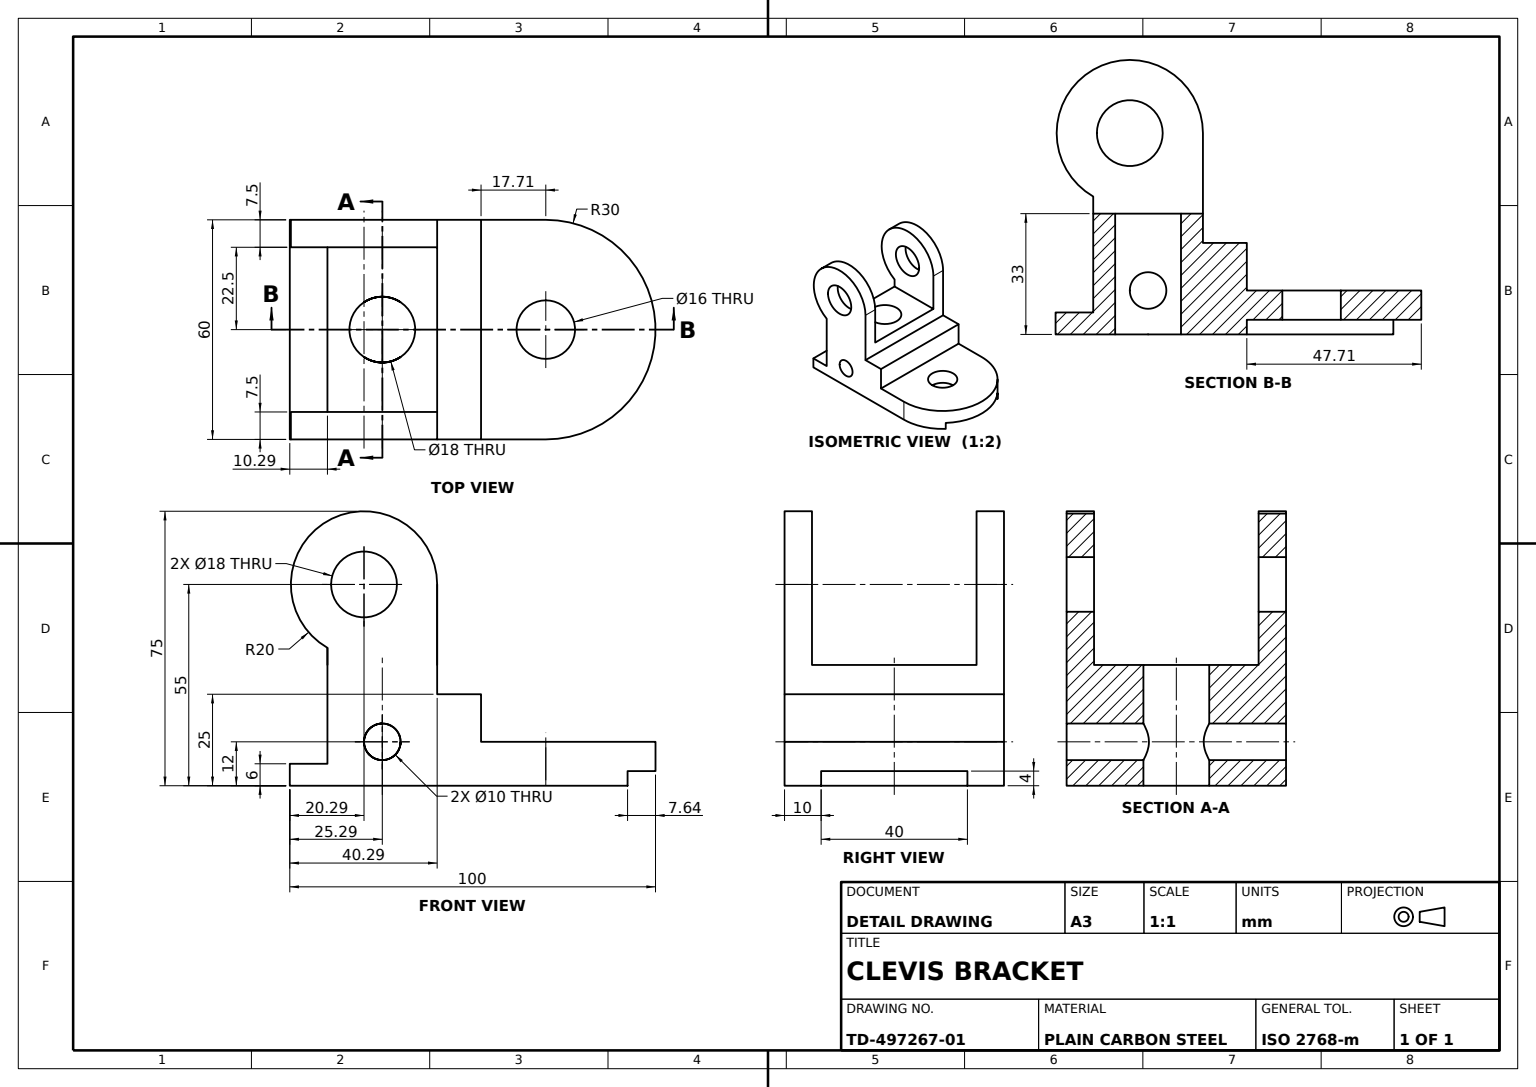
ISO-10303-21;
HEADER;
FILE_DESCRIPTION((''),'2;1');
FILE_NAME('','',(''),(''),'','','');
FILE_SCHEMA(('AUTOMOTIVE_DESIGN'));
ENDSEC;
DATA;
#1=APPLICATION_CONTEXT('');
#2=PRODUCT_CONTEXT('',#1,'mechanical');
#3=PRODUCT('','','',(#2));
#4=PRODUCT_DEFINITION_FORMATION('','',#3);
#5=PRODUCT_DEFINITION_CONTEXT('',#1,'design');
#6=PRODUCT_DEFINITION('','',#4,#5);
#7=PRODUCT_DEFINITION_SHAPE('','',#6);
#8=(LENGTH_UNIT()NAMED_UNIT(*)SI_UNIT(.MILLI.,.METRE.));
#9=(NAMED_UNIT(*)PLANE_ANGLE_UNIT()SI_UNIT($,.RADIAN.));
#10=(NAMED_UNIT(*)SI_UNIT($,.STERADIAN.)SOLID_ANGLE_UNIT());
#11=UNCERTAINTY_MEASURE_WITH_UNIT(LENGTH_MEASURE(1.E-05),#8,'distance_accuracy_value','');
#12=(GEOMETRIC_REPRESENTATION_CONTEXT(3)GLOBAL_UNCERTAINTY_ASSIGNED_CONTEXT((#11))GLOBAL_UNIT_ASSIGNED_CONTEXT((#8,#9,#10))REPRESENTATION_CONTEXT('',''));
#13=CARTESIAN_POINT('',(-9.705549,55.,-22.5));
#14=VERTEX_POINT('',#13);
#15=CARTESIAN_POINT('',(-9.705549,33.,-22.5));
#16=VERTEX_POINT('',#15);
#17=DIRECTION('',(0.,-1.,0.));
#18=VECTOR('',#17,1000.);
#19=LINE('',#13,#18);
#20=EDGE_CURVE('',#14,#16,#19,.T.);
#21=ORIENTED_EDGE('',*,*,#20,.T.);
#22=CARTESIAN_POINT('',(-9.705549,33.,22.5));
#23=VERTEX_POINT('',#22);
#24=CARTESIAN_POINT('',(-9.705549,33.,-30.));
#25=DIRECTION('',(0.,0.,1.));
#26=VECTOR('',#25,1000.);
#27=LINE('',#24,#26);
#28=EDGE_CURVE('',#16,#23,#27,.T.);
#29=ORIENTED_EDGE('',*,*,#28,.T.);
#30=CARTESIAN_POINT('',(-9.705549,55.,22.5));
#31=VERTEX_POINT('',#30);
#32=DIRECTION('',(0.,1.,0.));
#33=VECTOR('',#32,1000.);
#34=LINE('',#30,#33);
#35=EDGE_CURVE('',#23,#31,#34,.T.);
#36=ORIENTED_EDGE('',*,*,#35,.T.);
#37=CARTESIAN_POINT('',(-9.705549,55.,30.));
#38=VERTEX_POINT('',#37);
#39=LINE('',#30,#26);
#40=EDGE_CURVE('',#31,#38,#39,.T.);
#41=ORIENTED_EDGE('',*,*,#40,.T.);
#42=CARTESIAN_POINT('',(-9.705549,25.,30.));
#43=VERTEX_POINT('',#42);
#44=CARTESIAN_POINT('',(-9.705549,0.,30.));
#45=LINE('',#44,#33);
#46=EDGE_CURVE('',#43,#38,#45,.T.);
#47=ORIENTED_EDGE('',*,*,#46,.F.);
#48=CARTESIAN_POINT('',(-9.705549,25.,-30.));
#49=VERTEX_POINT('',#48);
#50=LINE('',#48,#26);
#51=EDGE_CURVE('',#49,#43,#50,.T.);
#52=ORIENTED_EDGE('',*,*,#51,.F.);
#53=CARTESIAN_POINT('',(-9.705549,55.,-30.));
#54=VERTEX_POINT('',#53);
#55=CARTESIAN_POINT('',(-9.705549,0.,-30.));
#56=LINE('',#55,#33);
#57=EDGE_CURVE('',#49,#54,#56,.T.);
#58=ORIENTED_EDGE('',*,*,#57,.T.);
#59=DIRECTION('',(0.,0.,-1.));
#60=VECTOR('',#59,1000.);
#61=LINE('',#13,#60);
#62=EDGE_CURVE('',#14,#54,#61,.T.);
#63=ORIENTED_EDGE('',*,*,#62,.F.);
#64=EDGE_LOOP('',(#21,#29,#36,#41,#47,#52,#58,#63));
#65=FACE_OUTER_BOUND('',#64,.T.);
#66=DIRECTION('',(1.,0.,0.));
#67=AXIS2_PLACEMENT_3D('',#55,#66,#59);
#68=PLANE('',#67);
#69=ADVANCED_FACE('',(#65),#68,.T.);
#70=CARTESIAN_POINT('',(2.294451,12.,30.));
#71=VERTEX_POINT('',#70);
#72=CARTESIAN_POINT('',(20.,12.,30.));
#73=VERTEX_POINT('',#72);
#74=VECTOR('',#66,1000.);
#75=LINE('',#70,#74);
#76=EDGE_CURVE('',#71,#73,#75,.T.);
#77=ORIENTED_EDGE('',*,*,#76,.T.);
#78=CARTESIAN_POINT('',(20.,12.,-30.));
#79=VERTEX_POINT('',#78);
#80=CARTESIAN_POINT('',(20.,12.,0.));
#81=AXIS2_PLACEMENT_3D('',#80,#32,#59);
#82=CIRCLE('',#81,30.);
#83=EDGE_CURVE('',#73,#79,#82,.T.);
#84=ORIENTED_EDGE('',*,*,#83,.T.);
#85=CARTESIAN_POINT('',(2.294451,12.,-30.));
#86=VERTEX_POINT('',#85);
#87=DIRECTION('',(-1.,0.,0.));
#88=VECTOR('',#87,1000.);
#89=LINE('',#78,#88);
#90=EDGE_CURVE('',#79,#86,#89,.T.);
#91=ORIENTED_EDGE('',*,*,#90,.T.);
#92=LINE('',#85,#26);
#93=EDGE_CURVE('',#86,#71,#92,.T.);
#94=ORIENTED_EDGE('',*,*,#93,.T.);
#95=EDGE_LOOP('',(#77,#84,#91,#94));
#96=FACE_OUTER_BOUND('',#95,.T.);
#97=CARTESIAN_POINT('',(20.,12.,8.));
#98=VERTEX_POINT('',#97);
#99=CARTESIAN_POINT('',(20.,12.,-8.));
#100=VERTEX_POINT('',#99);
#101=AXIS2_PLACEMENT_3D('',#80,#32,#25);
#102=CIRCLE('',#101,8.);
#103=EDGE_CURVE('',#98,#100,#102,.T.);
#104=ORIENTED_EDGE('',*,*,#103,.F.);
#105=EDGE_CURVE('',#100,#98,#102,.T.);
#106=ORIENTED_EDGE('',*,*,#105,.F.);
#107=EDGE_LOOP('',(#104,#106));
#108=FACE_BOUND('',#107,.T.);
#109=AXIS2_PLACEMENT_3D('',#80,#17,#59);
#110=PLANE('',#109);
#111=ADVANCED_FACE('',(#96,#108),#110,.F.);
#112=CARTESIAN_POINT('',(-39.705549,33.,22.5));
#113=VERTEX_POINT('',#112);
#114=LINE('',#112,#74);
#115=EDGE_CURVE('',#113,#23,#114,.T.);
#116=ORIENTED_EDGE('',*,*,#115,.T.);
#117=ORIENTED_EDGE('',*,*,#28,.F.);
#118=CARTESIAN_POINT('',(-39.705549,33.,-22.5));
#119=VERTEX_POINT('',#118);
#120=LINE('',#118,#88);
#121=EDGE_CURVE('',#16,#119,#120,.T.);
#122=ORIENTED_EDGE('',*,*,#121,.T.);
#123=CARTESIAN_POINT('',(-39.705549,33.,-30.));
#124=LINE('',#123,#26);
#125=EDGE_CURVE('',#119,#113,#124,.T.);
#126=ORIENTED_EDGE('',*,*,#125,.T.);
#127=EDGE_LOOP('',(#116,#117,#122,#126));
#128=FACE_OUTER_BOUND('',#127,.T.);
#129=CARTESIAN_POINT('',(-24.705549,33.,9.));
#130=VERTEX_POINT('',#129);
#131=CARTESIAN_POINT('',(-24.705549,33.,-9.));
#132=VERTEX_POINT('',#131);
#133=CARTESIAN_POINT('',(-24.705549,33.,0.));
#134=AXIS2_PLACEMENT_3D('',#133,#32,#25);
#135=CIRCLE('',#134,9.);
#136=EDGE_CURVE('',#130,#132,#135,.T.);
#137=ORIENTED_EDGE('',*,*,#136,.F.);
#138=EDGE_CURVE('',#132,#130,#135,.T.);
#139=ORIENTED_EDGE('',*,*,#138,.F.);
#140=EDGE_LOOP('',(#137,#139));
#141=FACE_BOUND('',#140,.T.);
#142=AXIS2_PLACEMENT_3D('',#123,#32,#25);
#143=PLANE('',#142);
#144=ADVANCED_FACE('',(#128,#141),#143,.T.);
#145=CARTESIAN_POINT('',(20.,4.,-8.));
#146=VERTEX_POINT('',#145);
#147=CARTESIAN_POINT('',(20.,0.,-8.));
#148=LINE('',#147,#33);
#149=EDGE_CURVE('',#146,#100,#148,.T.);
#150=ORIENTED_EDGE('',*,*,#149,.F.);
#151=CARTESIAN_POINT('',(20.,4.,8.));
#152=VERTEX_POINT('',#151);
#153=CARTESIAN_POINT('',(20.,4.,0.));
#154=AXIS2_PLACEMENT_3D('',#153,#32,#59);
#155=CIRCLE('',#154,8.);
#156=EDGE_CURVE('',#152,#146,#155,.T.);
#157=ORIENTED_EDGE('',*,*,#156,.F.);
#158=CARTESIAN_POINT('',(20.,0.,8.));
#159=LINE('',#158,#33);
#160=EDGE_CURVE('',#152,#98,#159,.T.);
#161=ORIENTED_EDGE('',*,*,#160,.T.);
#162=ORIENTED_EDGE('',*,*,#103,.T.);
#163=EDGE_LOOP('',(#150,#157,#161,#162));
#164=FACE_OUTER_BOUND('',#163,.T.);
#165=CARTESIAN_POINT('',(20.,0.,0.));
#166=AXIS2_PLACEMENT_3D('',#165,#32,#25);
#167=CYLINDRICAL_SURFACE('',#166,8.);
#168=ADVANCED_FACE('',(#164),#167,.F.);
#169=CARTESIAN_POINT('',(-38.705549,55.,22.5));
#170=VERTEX_POINT('',#169);
#171=CARTESIAN_POINT('',(-20.705549,55.,22.5));
#172=VERTEX_POINT('',#171);
#173=CARTESIAN_POINT('',(-29.705549,55.,22.5));
#174=AXIS2_PLACEMENT_3D('',#173,#25,#66);
#175=CIRCLE('',#174,9.);
#176=EDGE_CURVE('',#170,#172,#175,.T.);
#177=ORIENTED_EDGE('',*,*,#176,.F.);
#178=CARTESIAN_POINT('',(-38.705549,55.,30.));
#179=VERTEX_POINT('',#178);
#180=LINE('',#169,#26);
#181=EDGE_CURVE('',#170,#179,#180,.T.);
#182=ORIENTED_EDGE('',*,*,#181,.T.);
#183=CARTESIAN_POINT('',(-20.705549,55.,30.));
#184=VERTEX_POINT('',#183);
#185=CARTESIAN_POINT('',(-29.705549,55.,30.));
#186=AXIS2_PLACEMENT_3D('',#185,#25,#66);
#187=CIRCLE('',#186,9.);
#188=EDGE_CURVE('',#179,#184,#187,.T.);
#189=ORIENTED_EDGE('',*,*,#188,.T.);
#190=LINE('',#171,#26);
#191=EDGE_CURVE('',#172,#184,#190,.T.);
#192=ORIENTED_EDGE('',*,*,#191,.F.);
#193=EDGE_LOOP('',(#177,#182,#189,#192));
#194=FACE_OUTER_BOUND('',#193,.T.);
#195=CYLINDRICAL_SURFACE('',#174,9.);
#196=ADVANCED_FACE('',(#194),#195,.F.);
#197=CARTESIAN_POINT('',(-50.,6.,-30.));
#198=VERTEX_POINT('',#197);
#199=CARTESIAN_POINT('',(-50.,6.,30.));
#200=VERTEX_POINT('',#199);
#201=LINE('',#197,#26);
#202=EDGE_CURVE('',#198,#200,#201,.T.);
#203=ORIENTED_EDGE('',*,*,#202,.F.);
#204=CARTESIAN_POINT('',(-50.,0.,-30.));
#205=VERTEX_POINT('',#204);
#206=LINE('',#197,#18);
#207=EDGE_CURVE('',#198,#205,#206,.T.);
#208=ORIENTED_EDGE('',*,*,#207,.T.);
#209=CARTESIAN_POINT('',(-50.,0.,30.));
#210=VERTEX_POINT('',#209);
#211=LINE('',#204,#26);
#212=EDGE_CURVE('',#205,#210,#211,.T.);
#213=ORIENTED_EDGE('',*,*,#212,.T.);
#214=LINE('',#199,#18);
#215=EDGE_CURVE('',#200,#210,#214,.T.);
#216=ORIENTED_EDGE('',*,*,#215,.F.);
#217=EDGE_LOOP('',(#203,#208,#213,#216));
#218=FACE_OUTER_BOUND('',#217,.T.);
#219=AXIS2_PLACEMENT_3D('',#197,#66,#59);
#220=PLANE('',#219);
#221=ADVANCED_FACE('',(#218),#220,.F.);
#222=CARTESIAN_POINT('',(-49.705549,55.,-22.5));
#223=VERTEX_POINT('',#222);
#224=CARTESIAN_POINT('',(-49.705549,55.,-30.));
#225=VERTEX_POINT('',#224);
#226=LINE('',#222,#60);
#227=EDGE_CURVE('',#223,#225,#226,.T.);
#228=ORIENTED_EDGE('',*,*,#227,.F.);
#229=CARTESIAN_POINT('',(-29.705549,55.,-22.5));
#230=AXIS2_PLACEMENT_3D('',#229,#59,#87);
#231=CIRCLE('',#230,20.);
#232=EDGE_CURVE('',#223,#14,#231,.T.);
#233=ORIENTED_EDGE('',*,*,#232,.T.);
#234=ORIENTED_EDGE('',*,*,#62,.T.);
#235=CARTESIAN_POINT('',(-29.705549,55.,-30.));
#236=AXIS2_PLACEMENT_3D('',#235,#59,#87);
#237=CIRCLE('',#236,20.);
#238=EDGE_CURVE('',#225,#54,#237,.T.);
#239=ORIENTED_EDGE('',*,*,#238,.F.);
#240=EDGE_LOOP('',(#228,#233,#234,#239));
#241=FACE_OUTER_BOUND('',#240,.T.);
#242=CYLINDRICAL_SURFACE('',#230,20.);
#243=ADVANCED_FACE('',(#241),#242,.T.);
#244=ORIENTED_EDGE('',*,*,#227,.T.);
#245=CARTESIAN_POINT('',(-39.705549,37.679492,-30.));
#246=VERTEX_POINT('',#245);
#247=EDGE_CURVE('',#246,#225,#237,.T.);
#248=ORIENTED_EDGE('',*,*,#247,.F.);
#249=CARTESIAN_POINT('',(-39.705549,37.679492,-22.5));
#250=VERTEX_POINT('',#249);
#251=LINE('',#249,#60);
#252=EDGE_CURVE('',#250,#246,#251,.T.);
#253=ORIENTED_EDGE('',*,*,#252,.F.);
#254=EDGE_CURVE('',#250,#223,#231,.T.);
#255=ORIENTED_EDGE('',*,*,#254,.T.);
#256=EDGE_LOOP('',(#244,#248,#253,#255));
#257=FACE_OUTER_BOUND('',#256,.T.);
#258=ADVANCED_FACE('',(#257),#242,.T.);
#259=ORIENTED_EDGE('',*,*,#191,.T.);
#260=EDGE_CURVE('',#184,#179,#187,.T.);
#261=ORIENTED_EDGE('',*,*,#260,.T.);
#262=ORIENTED_EDGE('',*,*,#181,.F.);
#263=EDGE_CURVE('',#172,#170,#175,.T.);
#264=ORIENTED_EDGE('',*,*,#263,.F.);
#265=EDGE_LOOP('',(#259,#261,#262,#264));
#266=FACE_OUTER_BOUND('',#265,.T.);
#267=ADVANCED_FACE('',(#266),#195,.F.);
#268=ORIENTED_EDGE('',*,*,#156,.T.);
#269=EDGE_CURVE('',#146,#152,#155,.T.);
#270=ORIENTED_EDGE('',*,*,#269,.T.);
#271=EDGE_LOOP('',(#268,#270));
#272=FACE_BOUND('',#271,.T.);
#273=CARTESIAN_POINT('',(42.36068,4.,-20.));
#274=VERTEX_POINT('',#273);
#275=CARTESIAN_POINT('',(2.294451,4.,-20.));
#276=VERTEX_POINT('',#275);
#277=CARTESIAN_POINT('',(62.294451,4.,-20.));
#278=LINE('',#277,#88);
#279=EDGE_CURVE('',#274,#276,#278,.T.);
#280=ORIENTED_EDGE('',*,*,#279,.F.);
#281=CARTESIAN_POINT('',(42.36068,4.,20.));
#282=VERTEX_POINT('',#281);
#283=CIRCLE('',#154,30.);
#284=EDGE_CURVE('',#282,#274,#283,.T.);
#285=ORIENTED_EDGE('',*,*,#284,.F.);
#286=CARTESIAN_POINT('',(2.294451,4.,20.));
#287=VERTEX_POINT('',#286);
#288=CARTESIAN_POINT('',(62.294451,4.,20.));
#289=LINE('',#288,#88);
#290=EDGE_CURVE('',#282,#287,#289,.T.);
#291=ORIENTED_EDGE('',*,*,#290,.T.);
#292=LINE('',#286,#26);
#293=EDGE_CURVE('',#276,#287,#292,.T.);
#294=ORIENTED_EDGE('',*,*,#293,.F.);
#295=EDGE_LOOP('',(#280,#285,#291,#294));
#296=FACE_OUTER_BOUND('',#295,.T.);
#297=AXIS2_PLACEMENT_3D('',#288,#17,#59);
#298=PLANE('',#297);
#299=ADVANCED_FACE('',(#272,#296),#298,.T.);
#300=CARTESIAN_POINT('',(20.,0.,-30.));
#301=VERTEX_POINT('',#300);
#302=CARTESIAN_POINT('',(42.36068,0.,-20.));
#303=VERTEX_POINT('',#302);
#304=AXIS2_PLACEMENT_3D('',#165,#17,#25);
#305=CIRCLE('',#304,30.);
#306=EDGE_CURVE('',#301,#303,#305,.T.);
#307=ORIENTED_EDGE('',*,*,#306,.T.);
#308=CARTESIAN_POINT('',(2.294451,0.,-20.));
#309=VERTEX_POINT('',#308);
#310=CARTESIAN_POINT('',(62.294451,0.,-20.));
#311=LINE('',#310,#88);
#312=EDGE_CURVE('',#303,#309,#311,.T.);
#313=ORIENTED_EDGE('',*,*,#312,.T.);
#314=CARTESIAN_POINT('',(2.294451,0.,20.));
#315=VERTEX_POINT('',#314);
#316=LINE('',#314,#60);
#317=EDGE_CURVE('',#315,#309,#316,.T.);
#318=ORIENTED_EDGE('',*,*,#317,.F.);
#319=CARTESIAN_POINT('',(42.36068,0.,20.));
#320=VERTEX_POINT('',#319);
#321=CARTESIAN_POINT('',(62.294451,0.,20.));
#322=LINE('',#321,#88);
#323=EDGE_CURVE('',#320,#315,#322,.T.);
#324=ORIENTED_EDGE('',*,*,#323,.F.);
#325=CARTESIAN_POINT('',(20.,0.,30.));
#326=VERTEX_POINT('',#325);
#327=EDGE_CURVE('',#320,#326,#305,.T.);
#328=ORIENTED_EDGE('',*,*,#327,.T.);
#329=LINE('',#209,#74);
#330=EDGE_CURVE('',#210,#326,#329,.T.);
#331=ORIENTED_EDGE('',*,*,#330,.F.);
#332=ORIENTED_EDGE('',*,*,#212,.F.);
#333=LINE('',#204,#88);
#334=EDGE_CURVE('',#301,#205,#333,.T.);
#335=ORIENTED_EDGE('',*,*,#334,.F.);
#336=EDGE_LOOP('',(#307,#313,#318,#324,#328,#331,#332,#335));
#337=FACE_OUTER_BOUND('',#336,.T.);
#338=CARTESIAN_POINT('',(-24.705549,0.,-9.));
#339=VERTEX_POINT('',#338);
#340=CARTESIAN_POINT('',(-24.705549,0.,9.));
#341=VERTEX_POINT('',#340);
#342=CARTESIAN_POINT('',(-24.705549,0.,0.));
#343=AXIS2_PLACEMENT_3D('',#342,#32,#25);
#344=CIRCLE('',#343,9.);
#345=EDGE_CURVE('',#339,#341,#344,.T.);
#346=ORIENTED_EDGE('',*,*,#345,.T.);
#347=EDGE_CURVE('',#341,#339,#344,.T.);
#348=ORIENTED_EDGE('',*,*,#347,.T.);
#349=EDGE_LOOP('',(#346,#348));
#350=FACE_BOUND('',#349,.T.);
#351=CARTESIAN_POINT('',(0.,0.,0.));
#352=AXIS2_PLACEMENT_3D('',#351,#32,#25);
#353=PLANE('',#352);
#354=ADVANCED_FACE('',(#337,#350),#353,.F.);
#355=CARTESIAN_POINT('',(42.36068,6.,-20.));
#356=LINE('',#355,#18);
#357=EDGE_CURVE('',#274,#303,#356,.T.);
#358=ORIENTED_EDGE('',*,*,#357,.F.);
#359=ORIENTED_EDGE('',*,*,#279,.T.);
#360=LINE('',#308,#33);
#361=EDGE_CURVE('',#309,#276,#360,.T.);
#362=ORIENTED_EDGE('',*,*,#361,.F.);
#363=ORIENTED_EDGE('',*,*,#312,.F.);
#364=EDGE_LOOP('',(#358,#359,#362,#363));
#365=FACE_OUTER_BOUND('',#364,.T.);
#366=AXIS2_PLACEMENT_3D('',#310,#25,#66);
#367=PLANE('',#366);
#368=ADVANCED_FACE('',(#365),#367,.T.);
#369=CARTESIAN_POINT('',(-39.705549,37.679492,22.5));
#370=VERTEX_POINT('',#369);
#371=CIRCLE('',#174,20.);
#372=EDGE_CURVE('',#31,#370,#371,.T.);
#373=ORIENTED_EDGE('',*,*,#372,.F.);
#374=ORIENTED_EDGE('',*,*,#35,.F.);
#375=ORIENTED_EDGE('',*,*,#115,.F.);
#376=CARTESIAN_POINT('',(-39.705549,30.000541,22.5));
#377=LINE('',#376,#18);
#378=EDGE_CURVE('',#370,#113,#377,.T.);
#379=ORIENTED_EDGE('',*,*,#378,.F.);
#380=EDGE_LOOP('',(#373,#374,#375,#379));
#381=FACE_OUTER_BOUND('',#380,.T.);
#382=ORIENTED_EDGE('',*,*,#176,.T.);
#383=ORIENTED_EDGE('',*,*,#263,.T.);
#384=EDGE_LOOP('',(#382,#383));
#385=FACE_BOUND('',#384,.T.);
#386=PLANE('',#174);
#387=ADVANCED_FACE('',(#381,#385),#386,.F.);
#388=CARTESIAN_POINT('',(-19.705549,12.,-30.));
#389=VERTEX_POINT('',#388);
#390=CARTESIAN_POINT('',(-29.705549,12.,-30.));
#391=VERTEX_POINT('',#390);
#392=CARTESIAN_POINT('',(-24.705549,12.,-30.));
#393=AXIS2_PLACEMENT_3D('',#392,#25,#66);
#394=CIRCLE('',#393,5.);
#395=EDGE_CURVE('',#389,#391,#394,.T.);
#396=ORIENTED_EDGE('',*,*,#395,.F.);
#397=CARTESIAN_POINT('',(-19.705549,12.,-7.483315));
#398=VERTEX_POINT('',#397);
#399=LINE('',#388,#26);
#400=EDGE_CURVE('',#389,#398,#399,.T.);
#401=ORIENTED_EDGE('',*,*,#400,.T.);
#402=CARTESIAN_POINT('',(-24.705549,17.,-9.));
#403=VERTEX_POINT('',#402);
#404=CARTESIAN_POINT('',(-19.705549,12.338536,-7.483315));
#405=CARTESIAN_POINT('',(-19.739553,12.669551,-7.506333));
#406=CARTESIAN_POINT('',(-19.871033,13.317903,-7.59168));
#407=CARTESIAN_POINT('',(-19.970249,13.638042,-7.654971));
#408=CARTESIAN_POINT('',(-20.223004,14.238982,-7.805667));
#409=CARTESIAN_POINT('',(-20.376557,14.522849,-7.893121));
#410=CARTESIAN_POINT('',(-20.738291,15.06036,-8.08099));
#411=CARTESIAN_POINT('',(-20.942408,15.307695,-8.179185));
#412=CARTESIAN_POINT('',(-21.281111,15.646744,-8.323959));
#413=CARTESIAN_POINT('',(-21.399599,15.754555,-8.37188));
#414=CARTESIAN_POINT('',(-21.648313,15.959709,-8.465872));
#415=CARTESIAN_POINT('',(-21.779025,16.05729,-8.512072));
#416=CARTESIAN_POINT('',(-22.181396,16.328189,-8.643395));
#417=CARTESIAN_POINT('',(-22.465386,16.481988,-8.72219));
#418=CARTESIAN_POINT('',(-23.067114,16.735195,-8.854968));
#419=CARTESIAN_POINT('',(-23.389259,16.835025,-8.909233));
#420=CARTESIAN_POINT('',(-24.039683,16.966559,-8.981296));
#421=CARTESIAN_POINT('',(-24.369966,17.,-9.));
#422=B_SPLINE_CURVE_WITH_KNOTS('',3,(#397,#404,#405,#406,#407,#408,#409,#410,#411,#412,#413,#414,#415,#416,#417,#418,#419,#420,#421,#402),.UNSPECIFIED.,.F.,.F.,(4,2,2,2,2,2,2,2,2,4),(0.,0.000998979,0.001997959,0.002996938,0.003995917,0.004495407,0.004994896,0.005993876,0.006992855,0.007991834),.UNSPECIFIED.);
#423=EDGE_CURVE('',#398,#403,#422,.T.);
#424=ORIENTED_EDGE('',*,*,#423,.T.);
#425=CARTESIAN_POINT('',(-29.705549,12.,-7.483315));
#426=VERTEX_POINT('',#425);
#427=CARTESIAN_POINT('',(-24.873181,17.,-9.));
#428=CARTESIAN_POINT('',(-25.042873,16.991417,-8.995223));
#429=CARTESIAN_POINT('',(-25.375993,16.957674,-8.976544));
#430=CARTESIAN_POINT('',(-25.540439,16.932588,-8.962682));
#431=CARTESIAN_POINT('',(-25.86526,16.866471,-8.926465));
#432=CARTESIAN_POINT('',(-26.025633,16.825439,-8.904109));
#433=CARTESIAN_POINT('',(-26.342353,16.727405,-8.851364));
#434=CARTESIAN_POINT('',(-26.499142,16.670122,-8.820832));
#435=CARTESIAN_POINT('',(-26.953413,16.478301,-8.720282));
#436=CARTESIAN_POINT('',(-27.238345,16.323192,-8.640877));
#437=CARTESIAN_POINT('',(-27.775265,15.960036,-8.465025));
#438=CARTESIAN_POINT('',(-28.024927,15.75283,-8.369097));
#439=CARTESIAN_POINT('',(-28.475428,15.300002,-8.176067));
#440=CARTESIAN_POINT('',(-28.679659,15.051387,-8.077598));
#441=CARTESIAN_POINT('',(-29.039504,14.514228,-7.890372));
#442=CARTESIAN_POINT('',(-29.191838,14.231176,-7.803491));
#443=CARTESIAN_POINT('',(-29.379627,13.78304,-7.691444));
#444=CARTESIAN_POINT('',(-29.435378,13.629704,-7.657154));
#445=CARTESIAN_POINT('',(-29.532516,13.314384,-7.596294));
#446=CARTESIAN_POINT('',(-29.57396,13.151591,-7.569684));
#447=CARTESIAN_POINT('',(-29.672498,12.663149,-7.505701));
#448=CARTESIAN_POINT('',(-29.705549,12.333608,-7.483315));
#449=B_SPLINE_CURVE_WITH_KNOTS('',3,(#402,#427,#428,#429,#430,#431,#432,#433,#434,#435,#436,#437,#438,#439,#440,#441,#442,#443,#444,#445,#446,#447,#448,#425),.UNSPECIFIED.,.F.,.F.,(4,2,2,2,2,2,2,2,2,2,2,4),(0.007991834,0.008490847,0.00898986,0.009488874,0.009987887,0.010985913,0.011983939,0.012981966,0.013979992,0.014479005,0.014978018,0.015976045),.UNSPECIFIED.);
#450=EDGE_CURVE('',#403,#426,#449,.T.);
#451=ORIENTED_EDGE('',*,*,#450,.T.);
#452=LINE('',#390,#26);
#453=EDGE_CURVE('',#391,#426,#452,.T.);
#454=ORIENTED_EDGE('',*,*,#453,.F.);
#455=EDGE_LOOP('',(#396,#401,#424,#451,#454));
#456=FACE_OUTER_BOUND('',#455,.T.);
#457=CYLINDRICAL_SURFACE('',#393,5.);
#458=ADVANCED_FACE('',(#456),#457,.F.);
#459=CARTESIAN_POINT('',(-38.705549,55.,-30.));
#460=VERTEX_POINT('',#459);
#461=CARTESIAN_POINT('',(-20.705549,55.,-30.));
#462=VERTEX_POINT('',#461);
#463=CIRCLE('',#236,9.);
#464=EDGE_CURVE('',#460,#462,#463,.T.);
#465=ORIENTED_EDGE('',*,*,#464,.T.);
#466=CARTESIAN_POINT('',(-20.705549,55.,-22.5));
#467=VERTEX_POINT('',#466);
#468=LINE('',#466,#60);
#469=EDGE_CURVE('',#467,#462,#468,.T.);
#470=ORIENTED_EDGE('',*,*,#469,.F.);
#471=CARTESIAN_POINT('',(-38.705549,55.,-22.5));
#472=VERTEX_POINT('',#471);
#473=CIRCLE('',#230,9.);
#474=EDGE_CURVE('',#472,#467,#473,.T.);
#475=ORIENTED_EDGE('',*,*,#474,.F.);
#476=LINE('',#471,#60);
#477=EDGE_CURVE('',#472,#460,#476,.T.);
#478=ORIENTED_EDGE('',*,*,#477,.T.);
#479=EDGE_LOOP('',(#465,#470,#475,#478));
#480=FACE_OUTER_BOUND('',#479,.T.);
#481=CYLINDRICAL_SURFACE('',#230,9.);
#482=ADVANCED_FACE('',(#480),#481,.F.);
#483=ORIENTED_EDGE('',*,*,#477,.F.);
#484=EDGE_CURVE('',#467,#472,#473,.T.);
#485=ORIENTED_EDGE('',*,*,#484,.F.);
#486=ORIENTED_EDGE('',*,*,#469,.T.);
#487=EDGE_CURVE('',#462,#460,#463,.T.);
#488=ORIENTED_EDGE('',*,*,#487,.T.);
#489=EDGE_LOOP('',(#483,#485,#486,#488));
#490=FACE_OUTER_BOUND('',#489,.T.);
#491=ADVANCED_FACE('',(#490),#481,.F.);
#492=CARTESIAN_POINT('',(-24.705549,17.,9.));
#493=VERTEX_POINT('',#492);
#494=LINE('',#340,#33);
#495=EDGE_CURVE('',#493,#130,#494,.T.);
#496=ORIENTED_EDGE('',*,*,#495,.F.);
#497=CARTESIAN_POINT('',(-29.705549,12.,7.483315));
#498=VERTEX_POINT('',#497);
#499=CARTESIAN_POINT('',(-29.705549,12.333174,7.483315));
#500=CARTESIAN_POINT('',(-29.671185,12.672339,7.506574));
#501=CARTESIAN_POINT('',(-29.539208,13.321106,7.592228));
#502=CARTESIAN_POINT('',(-29.440984,13.637996,7.654905));
#503=CARTESIAN_POINT('',(-29.186707,14.242007,7.80648));
#504=CARTESIAN_POINT('',(-29.032864,14.525482,7.894012));
#505=CARTESIAN_POINT('',(-28.673132,15.059738,8.080802));
#506=CARTESIAN_POINT('',(-28.466821,15.309793,8.180042));
#507=CARTESIAN_POINT('',(-28.015389,15.761231,8.372885));
#508=CARTESIAN_POINT('',(-27.768683,15.965245,8.46746));
#509=CARTESIAN_POINT('',(-27.22871,16.328928,8.643745));
#510=CARTESIAN_POINT('',(-26.942856,16.483334,8.722888));
#511=CARTESIAN_POINT('',(-26.493012,16.672412,8.822049));
#512=CARTESIAN_POINT('',(-26.339343,16.728418,8.851906));
#513=CARTESIAN_POINT('',(-26.024119,16.825825,8.904319));
#514=CARTESIAN_POINT('',(-25.861423,16.867437,8.926991));
#515=CARTESIAN_POINT('',(-25.369543,16.966996,8.981535));
#516=CARTESIAN_POINT('',(-25.038904,17.,9.));
#517=B_SPLINE_CURVE_WITH_KNOTS('',3,(#497,#499,#500,#501,#502,#503,#504,#505,#506,#507,#508,#509,#510,#511,#512,#513,#514,#515,#516,#492),.UNSPECIFIED.,.F.,.F.,(4,2,2,2,2,2,2,2,2,4),(0.015976045,0.016972773,0.017969501,0.018966229,0.019962957,0.020959685,0.021956413,0.022454777,0.022953141,0.023949869),.UNSPECIFIED.);
#518=EDGE_CURVE('',#498,#493,#517,.T.);
#519=ORIENTED_EDGE('',*,*,#518,.F.);
#520=CARTESIAN_POINT('',(-24.705549,7.,9.));
#521=VERTEX_POINT('',#520);
#522=CARTESIAN_POINT('',(-24.873181,7.,9.));
#523=CARTESIAN_POINT('',(-25.042873,7.008583,8.995223));
#524=CARTESIAN_POINT('',(-25.375993,7.042326,8.976544));
#525=CARTESIAN_POINT('',(-25.540439,7.067412,8.962682));
#526=CARTESIAN_POINT('',(-25.86526,7.133529,8.926465));
#527=CARTESIAN_POINT('',(-26.025633,7.174561,8.904109));
#528=CARTESIAN_POINT('',(-26.342353,7.272595,8.851364));
#529=CARTESIAN_POINT('',(-26.499142,7.329878,8.820832));
#530=CARTESIAN_POINT('',(-26.953413,7.521699,8.720282));
#531=CARTESIAN_POINT('',(-27.238345,7.676808,8.640877));
#532=CARTESIAN_POINT('',(-27.775265,8.039964,8.465025));
#533=CARTESIAN_POINT('',(-28.024927,8.24717,8.369097));
#534=CARTESIAN_POINT('',(-28.475428,8.699998,8.176067));
#535=CARTESIAN_POINT('',(-28.679659,8.948613,8.077598));
#536=CARTESIAN_POINT('',(-29.039504,9.485772,7.890372));
#537=CARTESIAN_POINT('',(-29.191838,9.768824,7.803491));
#538=CARTESIAN_POINT('',(-29.379627,10.21696,7.691444));
#539=CARTESIAN_POINT('',(-29.435378,10.370296,7.657154));
#540=CARTESIAN_POINT('',(-29.532516,10.685616,7.596294));
#541=CARTESIAN_POINT('',(-29.57396,10.848409,7.569684));
#542=CARTESIAN_POINT('',(-29.672498,11.336851,7.505701));
#543=CARTESIAN_POINT('',(-29.705549,11.666392,7.483315));
#544=B_SPLINE_CURVE_WITH_KNOTS('',3,(#520,#522,#523,#524,#525,#526,#527,#528,#529,#530,#531,#532,#533,#534,#535,#536,#537,#538,#539,#540,#541,#542,#543,#497),.UNSPECIFIED.,.F.,.F.,(4,2,2,2,2,2,2,2,2,2,2,4),(0.007991834,0.008490847,0.00898986,0.009488874,0.009987887,0.010985913,0.011983939,0.012981966,0.013979992,0.014479005,0.014978018,0.015976045),.UNSPECIFIED.);
#545=EDGE_CURVE('',#521,#498,#544,.T.);
#546=ORIENTED_EDGE('',*,*,#545,.F.);
#547=EDGE_CURVE('',#341,#521,#494,.T.);
#548=ORIENTED_EDGE('',*,*,#547,.F.);
#549=ORIENTED_EDGE('',*,*,#345,.F.);
#550=CARTESIAN_POINT('',(-24.705549,7.,-9.));
#551=VERTEX_POINT('',#550);
#552=LINE('',#338,#33);
#553=EDGE_CURVE('',#339,#551,#552,.T.);
#554=ORIENTED_EDGE('',*,*,#553,.T.);
#555=CARTESIAN_POINT('',(-29.705549,11.666826,-7.483315));
#556=CARTESIAN_POINT('',(-29.671185,11.327661,-7.506574));
#557=CARTESIAN_POINT('',(-29.539208,10.678894,-7.592228));
#558=CARTESIAN_POINT('',(-29.440984,10.362004,-7.654905));
#559=CARTESIAN_POINT('',(-29.186707,9.757993,-7.80648));
#560=CARTESIAN_POINT('',(-29.032864,9.474518,-7.894012));
#561=CARTESIAN_POINT('',(-28.673132,8.940262,-8.080802));
#562=CARTESIAN_POINT('',(-28.466821,8.690207,-8.180042));
#563=CARTESIAN_POINT('',(-28.015389,8.238769,-8.372885));
#564=CARTESIAN_POINT('',(-27.768683,8.034755,-8.46746));
#565=CARTESIAN_POINT('',(-27.22871,7.671072,-8.643745));
#566=CARTESIAN_POINT('',(-26.942856,7.516666,-8.722888));
#567=CARTESIAN_POINT('',(-26.493012,7.327588,-8.822049));
#568=CARTESIAN_POINT('',(-26.339343,7.271582,-8.851906));
#569=CARTESIAN_POINT('',(-26.024119,7.174175,-8.904319));
#570=CARTESIAN_POINT('',(-25.861423,7.132563,-8.926991));
#571=CARTESIAN_POINT('',(-25.369543,7.033004,-8.981535));
#572=CARTESIAN_POINT('',(-25.038904,7.,-9.));
#573=B_SPLINE_CURVE_WITH_KNOTS('',3,(#425,#555,#556,#557,#558,#559,#560,#561,#562,#563,#564,#565,#566,#567,#568,#569,#570,#571,#572,#550),.UNSPECIFIED.,.F.,.F.,(4,2,2,2,2,2,2,2,2,4),(0.015976045,0.016972773,0.017969501,0.018966229,0.019962957,0.020959685,0.021956413,0.022454777,0.022953141,0.023949869),.UNSPECIFIED.);
#574=EDGE_CURVE('',#426,#551,#573,.T.);
#575=ORIENTED_EDGE('',*,*,#574,.F.);
#576=ORIENTED_EDGE('',*,*,#450,.F.);
#577=EDGE_CURVE('',#403,#132,#552,.T.);
#578=ORIENTED_EDGE('',*,*,#577,.T.);
#579=ORIENTED_EDGE('',*,*,#138,.T.);
#580=EDGE_LOOP('',(#496,#519,#546,#548,#549,#554,#575,#576,#578,#579));
#581=FACE_OUTER_BOUND('',#580,.T.);
#582=CYLINDRICAL_SURFACE('',#343,9.);
#583=ADVANCED_FACE('',(#581),#582,.F.);
#584=ORIENTED_EDGE('',*,*,#51,.T.);
#585=CARTESIAN_POINT('',(2.294451,25.,30.));
#586=VERTEX_POINT('',#585);
#587=LINE('',#42,#88);
#588=EDGE_CURVE('',#586,#43,#587,.T.);
#589=ORIENTED_EDGE('',*,*,#588,.F.);
#590=CARTESIAN_POINT('',(2.294451,25.,-30.));
#591=VERTEX_POINT('',#590);
#592=LINE('',#590,#26);
#593=EDGE_CURVE('',#591,#586,#592,.T.);
#594=ORIENTED_EDGE('',*,*,#593,.F.);
#595=LINE('',#48,#88);
#596=EDGE_CURVE('',#591,#49,#595,.T.);
#597=ORIENTED_EDGE('',*,*,#596,.T.);
#598=EDGE_LOOP('',(#584,#589,#594,#597));
#599=FACE_OUTER_BOUND('',#598,.T.);
#600=AXIS2_PLACEMENT_3D('',#48,#32,#87);
#601=PLANE('',#600);
#602=ADVANCED_FACE('',(#599),#601,.T.);
#603=CARTESIAN_POINT('',(-39.705549,6.,-30.));
#604=VERTEX_POINT('',#603);
#605=LINE('',#197,#88);
#606=EDGE_CURVE('',#604,#198,#605,.T.);
#607=ORIENTED_EDGE('',*,*,#606,.F.);
#608=CARTESIAN_POINT('',(-39.705549,0.,-30.));
#609=LINE('',#608,#18);
#610=EDGE_CURVE('',#246,#604,#609,.T.);
#611=ORIENTED_EDGE('',*,*,#610,.F.);
#612=ORIENTED_EDGE('',*,*,#247,.T.);
#613=ORIENTED_EDGE('',*,*,#238,.T.);
#614=ORIENTED_EDGE('',*,*,#57,.F.);
#615=ORIENTED_EDGE('',*,*,#596,.F.);
#616=CARTESIAN_POINT('',(2.294451,0.,-30.));
#617=LINE('',#616,#33);
#618=EDGE_CURVE('',#86,#591,#617,.T.);
#619=ORIENTED_EDGE('',*,*,#618,.F.);
#620=ORIENTED_EDGE('',*,*,#90,.F.);
#621=CARTESIAN_POINT('',(20.,6.,-30.));
#622=LINE('',#621,#18);
#623=EDGE_CURVE('',#79,#301,#622,.T.);
#624=ORIENTED_EDGE('',*,*,#623,.T.);
#625=ORIENTED_EDGE('',*,*,#334,.T.);
#626=ORIENTED_EDGE('',*,*,#207,.F.);
#627=EDGE_LOOP('',(#607,#611,#612,#613,#614,#615,#619,#620,#624,#625,#626));
#628=FACE_OUTER_BOUND('',#627,.T.);
#629=ORIENTED_EDGE('',*,*,#487,.F.);
#630=ORIENTED_EDGE('',*,*,#464,.F.);
#631=EDGE_LOOP('',(#629,#630));
#632=FACE_BOUND('',#631,.T.);
#633=EDGE_CURVE('',#391,#389,#394,.T.);
#634=ORIENTED_EDGE('',*,*,#633,.T.);
#635=ORIENTED_EDGE('',*,*,#395,.T.);
#636=EDGE_LOOP('',(#634,#635));
#637=FACE_BOUND('',#636,.T.);
#638=AXIS2_PLACEMENT_3D('',#197,#25,#66);
#639=PLANE('',#638);
#640=ADVANCED_FACE('',(#628,#632,#637),#639,.F.);
#641=ORIENTED_EDGE('',*,*,#484,.T.);
#642=ORIENTED_EDGE('',*,*,#474,.T.);
#643=EDGE_LOOP('',(#641,#642));
#644=FACE_BOUND('',#643,.T.);
#645=ORIENTED_EDGE('',*,*,#20,.F.);
#646=ORIENTED_EDGE('',*,*,#232,.F.);
#647=ORIENTED_EDGE('',*,*,#254,.F.);
#648=CARTESIAN_POINT('',(-39.705549,28.623503,-22.5));
#649=LINE('',#648,#33);
#650=EDGE_CURVE('',#119,#250,#649,.T.);
#651=ORIENTED_EDGE('',*,*,#650,.F.);
#652=ORIENTED_EDGE('',*,*,#121,.F.);
#653=EDGE_LOOP('',(#645,#646,#647,#651,#652));
#654=FACE_OUTER_BOUND('',#653,.T.);
#655=PLANE('',#230);
#656=ADVANCED_FACE('',(#644,#654),#655,.F.);
#657=ORIENTED_EDGE('',*,*,#317,.T.);
#658=ORIENTED_EDGE('',*,*,#361,.T.);
#659=ORIENTED_EDGE('',*,*,#293,.T.);
#660=LINE('',#314,#18);
#661=EDGE_CURVE('',#287,#315,#660,.T.);
#662=ORIENTED_EDGE('',*,*,#661,.T.);
#663=EDGE_LOOP('',(#657,#658,#659,#662));
#664=FACE_OUTER_BOUND('',#663,.T.);
#665=CARTESIAN_POINT('',(2.294451,0.,0.));
#666=AXIS2_PLACEMENT_3D('',#665,#87,#25);
#667=PLANE('',#666);
#668=ADVANCED_FACE('',(#664),#667,.F.);
#669=CARTESIAN_POINT('',(-19.705549,12.,7.483315));
#670=VERTEX_POINT('',#669);
#671=CARTESIAN_POINT('',(-24.372766,17.,9.));
#672=CARTESIAN_POINT('',(-24.033945,16.965779,8.980863));
#673=CARTESIAN_POINT('',(-23.38389,16.833553,8.908433));
#674=CARTESIAN_POINT('',(-23.068701,16.736031,8.855396));
#675=CARTESIAN_POINT('',(-22.459478,16.479333,8.720807));
#676=CARTESIAN_POINT('',(-22.174678,16.324189,8.641395));
#677=CARTESIAN_POINT('',(-21.640364,15.963402,8.46662));
#678=CARTESIAN_POINT('',(-21.389446,15.755736,8.370403));
#679=CARTESIAN_POINT('',(-20.938348,15.303073,8.177309));
#680=CARTESIAN_POINT('',(-20.735928,15.057097,8.079797));
#681=CARTESIAN_POINT('',(-20.466369,14.656179,7.939748));
#682=CARTESIAN_POINT('',(-20.382071,14.516672,7.894002));
#683=CARTESIAN_POINT('',(-20.228608,14.232287,7.807992));
#684=CARTESIAN_POINT('',(-20.158959,14.086776,7.767486));
#685=CARTESIAN_POINT('',(-19.971081,13.639895,7.65546));
#686=CARTESIAN_POINT('',(-19.873628,13.328311,7.593346));
#687=CARTESIAN_POINT('',(-19.739759,12.672902,7.506483));
#688=CARTESIAN_POINT('',(-19.705549,12.337194,7.483315));
#689=B_SPLINE_CURVE_WITH_KNOTS('',3,(#492,#671,#672,#673,#674,#675,#676,#677,#678,#679,#680,#681,#682,#683,#684,#685,#686,#687,#688,#669),.UNSPECIFIED.,.F.,.F.,(4,2,2,2,2,2,2,2,2,4),(0.023949869,0.024944888,0.025939907,0.026934926,0.027929944,0.028924963,0.029422472,0.029919982,0.030915,0.031910019),.UNSPECIFIED.);
#690=EDGE_CURVE('',#493,#670,#689,.T.);
#691=ORIENTED_EDGE('',*,*,#690,.F.);
#692=ORIENTED_EDGE('',*,*,#495,.T.);
#693=ORIENTED_EDGE('',*,*,#136,.T.);
#694=ORIENTED_EDGE('',*,*,#577,.F.);
#695=ORIENTED_EDGE('',*,*,#423,.F.);
#696=CARTESIAN_POINT('',(-24.372766,7.,-9.));
#697=CARTESIAN_POINT('',(-24.033945,7.034221,-8.980863));
#698=CARTESIAN_POINT('',(-23.38389,7.166447,-8.908433));
#699=CARTESIAN_POINT('',(-23.068701,7.263969,-8.855396));
#700=CARTESIAN_POINT('',(-22.459478,7.520667,-8.720807));
#701=CARTESIAN_POINT('',(-22.174678,7.675811,-8.641395));
#702=CARTESIAN_POINT('',(-21.640364,8.036598,-8.46662));
#703=CARTESIAN_POINT('',(-21.389446,8.244264,-8.370403));
#704=CARTESIAN_POINT('',(-20.938348,8.696927,-8.177309));
#705=CARTESIAN_POINT('',(-20.735928,8.942903,-8.079797));
#706=CARTESIAN_POINT('',(-20.466369,9.343821,-7.939748));
#707=CARTESIAN_POINT('',(-20.382071,9.483328,-7.894002));
#708=CARTESIAN_POINT('',(-20.228608,9.767713,-7.807992));
#709=CARTESIAN_POINT('',(-20.158959,9.913224,-7.767486));
#710=CARTESIAN_POINT('',(-19.971081,10.360105,-7.65546));
#711=CARTESIAN_POINT('',(-19.873628,10.671689,-7.593346));
#712=CARTESIAN_POINT('',(-19.739759,11.327098,-7.506483));
#713=CARTESIAN_POINT('',(-19.705549,11.662806,-7.483315));
#714=B_SPLINE_CURVE_WITH_KNOTS('',3,(#550,#696,#697,#698,#699,#700,#701,#702,#703,#704,#705,#706,#707,#708,#709,#710,#711,#712,#713,#397),.UNSPECIFIED.,.F.,.F.,(4,2,2,2,2,2,2,2,2,4),(0.023949869,0.024944888,0.025939907,0.026934926,0.027929944,0.028924963,0.029422472,0.029919982,0.030915,0.031910019),.UNSPECIFIED.);
#715=EDGE_CURVE('',#551,#398,#714,.T.);
#716=ORIENTED_EDGE('',*,*,#715,.F.);
#717=ORIENTED_EDGE('',*,*,#553,.F.);
#718=ORIENTED_EDGE('',*,*,#347,.F.);
#719=ORIENTED_EDGE('',*,*,#547,.T.);
#720=CARTESIAN_POINT('',(-19.705549,11.661464,7.483315));
#721=CARTESIAN_POINT('',(-19.739553,11.330449,7.506333));
#722=CARTESIAN_POINT('',(-19.871033,10.682097,7.59168));
#723=CARTESIAN_POINT('',(-19.970249,10.361958,7.654971));
#724=CARTESIAN_POINT('',(-20.223004,9.761018,7.805667));
#725=CARTESIAN_POINT('',(-20.376557,9.477151,7.893121));
#726=CARTESIAN_POINT('',(-20.738291,8.93964,8.08099));
#727=CARTESIAN_POINT('',(-20.942408,8.692305,8.179185));
#728=CARTESIAN_POINT('',(-21.281111,8.353256,8.323959));
#729=CARTESIAN_POINT('',(-21.399599,8.245445,8.37188));
#730=CARTESIAN_POINT('',(-21.648313,8.040291,8.465872));
#731=CARTESIAN_POINT('',(-21.779025,7.94271,8.512072));
#732=CARTESIAN_POINT('',(-22.181396,7.671811,8.643395));
#733=CARTESIAN_POINT('',(-22.465386,7.518012,8.72219));
#734=CARTESIAN_POINT('',(-23.067114,7.264805,8.854968));
#735=CARTESIAN_POINT('',(-23.389259,7.164975,8.909233));
#736=CARTESIAN_POINT('',(-24.039683,7.033441,8.981296));
#737=CARTESIAN_POINT('',(-24.369966,7.,9.));
#738=B_SPLINE_CURVE_WITH_KNOTS('',3,(#669,#720,#721,#722,#723,#724,#725,#726,#727,#728,#729,#730,#731,#732,#733,#734,#735,#736,#737,#520),.UNSPECIFIED.,.F.,.F.,(4,2,2,2,2,2,2,2,2,4),(0.,0.000998979,0.001997959,0.002996938,0.003995917,0.004495407,0.004994896,0.005993876,0.006992855,0.007991834),.UNSPECIFIED.);
#739=EDGE_CURVE('',#670,#521,#738,.T.);
#740=ORIENTED_EDGE('',*,*,#739,.F.);
#741=EDGE_LOOP('',(#691,#692,#693,#694,#695,#716,#717,#718,#719,#740));
#742=FACE_OUTER_BOUND('',#741,.T.);
#743=ADVANCED_FACE('',(#742),#582,.F.);
#744=CARTESIAN_POINT('',(-29.705549,12.,30.));
#745=VERTEX_POINT('',#744);
#746=EDGE_CURVE('',#498,#745,#452,.T.);
#747=ORIENTED_EDGE('',*,*,#746,.T.);
#748=CARTESIAN_POINT('',(-19.705549,12.,30.));
#749=VERTEX_POINT('',#748);
#750=CARTESIAN_POINT('',(-24.705549,12.,30.));
#751=AXIS2_PLACEMENT_3D('',#750,#25,#66);
#752=CIRCLE('',#751,5.);
#753=EDGE_CURVE('',#745,#749,#752,.T.);
#754=ORIENTED_EDGE('',*,*,#753,.T.);
#755=EDGE_CURVE('',#670,#749,#399,.T.);
#756=ORIENTED_EDGE('',*,*,#755,.F.);
#757=ORIENTED_EDGE('',*,*,#739,.T.);
#758=ORIENTED_EDGE('',*,*,#545,.T.);
#759=EDGE_LOOP('',(#747,#754,#756,#757,#758));
#760=FACE_OUTER_BOUND('',#759,.T.);
#761=ADVANCED_FACE('',(#760),#457,.F.);
#762=ORIENTED_EDGE('',*,*,#650,.T.);
#763=ORIENTED_EDGE('',*,*,#252,.T.);
#764=ORIENTED_EDGE('',*,*,#610,.T.);
#765=CARTESIAN_POINT('',(-39.705549,6.,30.));
#766=VERTEX_POINT('',#765);
#767=CARTESIAN_POINT('',(-39.705549,6.,0.));
#768=LINE('',#767,#26);
#769=EDGE_CURVE('',#604,#766,#768,.T.);
#770=ORIENTED_EDGE('',*,*,#769,.T.);
#771=CARTESIAN_POINT('',(-39.705549,37.679492,30.));
#772=VERTEX_POINT('',#771);
#773=CARTESIAN_POINT('',(-39.705549,0.,30.));
#774=LINE('',#773,#18);
#775=EDGE_CURVE('',#772,#766,#774,.T.);
#776=ORIENTED_EDGE('',*,*,#775,.F.);
#777=LINE('',#369,#26);
#778=EDGE_CURVE('',#370,#772,#777,.T.);
#779=ORIENTED_EDGE('',*,*,#778,.F.);
#780=ORIENTED_EDGE('',*,*,#378,.T.);
#781=ORIENTED_EDGE('',*,*,#125,.F.);
#782=EDGE_LOOP('',(#762,#763,#764,#770,#776,#779,#780,#781));
#783=FACE_OUTER_BOUND('',#782,.T.);
#784=AXIS2_PLACEMENT_3D('',#608,#87,#25);
#785=PLANE('',#784);
#786=ADVANCED_FACE('',(#783),#785,.T.);
#787=ORIENTED_EDGE('',*,*,#574,.T.);
#788=ORIENTED_EDGE('',*,*,#715,.T.);
#789=ORIENTED_EDGE('',*,*,#400,.F.);
#790=ORIENTED_EDGE('',*,*,#633,.F.);
#791=ORIENTED_EDGE('',*,*,#453,.T.);
#792=EDGE_LOOP('',(#787,#788,#789,#790,#791));
#793=FACE_OUTER_BOUND('',#792,.T.);
#794=ADVANCED_FACE('',(#793),#457,.F.);
#795=CARTESIAN_POINT('',(42.36068,6.,20.));
#796=LINE('',#795,#33);
#797=EDGE_CURVE('',#320,#282,#796,.T.);
#798=ORIENTED_EDGE('',*,*,#797,.F.);
#799=ORIENTED_EDGE('',*,*,#323,.T.);
#800=ORIENTED_EDGE('',*,*,#661,.F.);
#801=ORIENTED_EDGE('',*,*,#290,.F.);
#802=EDGE_LOOP('',(#798,#799,#800,#801));
#803=FACE_OUTER_BOUND('',#802,.T.);
#804=AXIS2_PLACEMENT_3D('',#321,#59,#87);
#805=PLANE('',#804);
#806=ADVANCED_FACE('',(#803),#805,.T.);
#807=ORIENTED_EDGE('',*,*,#40,.F.);
#808=ORIENTED_EDGE('',*,*,#372,.T.);
#809=ORIENTED_EDGE('',*,*,#778,.T.);
#810=CIRCLE('',#186,20.);
#811=EDGE_CURVE('',#38,#772,#810,.T.);
#812=ORIENTED_EDGE('',*,*,#811,.F.);
#813=EDGE_LOOP('',(#807,#808,#809,#812));
#814=FACE_OUTER_BOUND('',#813,.T.);
#815=CYLINDRICAL_SURFACE('',#174,20.);
#816=ADVANCED_FACE('',(#814),#815,.T.);
#817=ORIENTED_EDGE('',*,*,#93,.F.);
#818=ORIENTED_EDGE('',*,*,#618,.T.);
#819=ORIENTED_EDGE('',*,*,#593,.T.);
#820=CARTESIAN_POINT('',(2.294451,0.,30.));
#821=LINE('',#820,#33);
#822=EDGE_CURVE('',#71,#586,#821,.T.);
#823=ORIENTED_EDGE('',*,*,#822,.F.);
#824=EDGE_LOOP('',(#817,#818,#819,#823));
#825=FACE_OUTER_BOUND('',#824,.T.);
#826=AXIS2_PLACEMENT_3D('',#616,#66,#59);
#827=PLANE('',#826);
#828=ADVANCED_FACE('',(#825),#827,.T.);
#829=EDGE_CURVE('',#749,#745,#752,.T.);
#830=ORIENTED_EDGE('',*,*,#829,.T.);
#831=ORIENTED_EDGE('',*,*,#746,.F.);
#832=ORIENTED_EDGE('',*,*,#518,.T.);
#833=ORIENTED_EDGE('',*,*,#690,.T.);
#834=ORIENTED_EDGE('',*,*,#755,.T.);
#835=EDGE_LOOP('',(#830,#831,#832,#833,#834));
#836=FACE_OUTER_BOUND('',#835,.T.);
#837=ADVANCED_FACE('',(#836),#457,.F.);
#838=ORIENTED_EDGE('',*,*,#160,.F.);
#839=ORIENTED_EDGE('',*,*,#269,.F.);
#840=ORIENTED_EDGE('',*,*,#149,.T.);
#841=ORIENTED_EDGE('',*,*,#105,.T.);
#842=EDGE_LOOP('',(#838,#839,#840,#841));
#843=FACE_OUTER_BOUND('',#842,.T.);
#844=ADVANCED_FACE('',(#843),#167,.F.);
#845=ORIENTED_EDGE('',*,*,#260,.F.);
#846=ORIENTED_EDGE('',*,*,#188,.F.);
#847=EDGE_LOOP('',(#845,#846));
#848=FACE_BOUND('',#847,.T.);
#849=ORIENTED_EDGE('',*,*,#829,.F.);
#850=ORIENTED_EDGE('',*,*,#753,.F.);
#851=EDGE_LOOP('',(#849,#850));
#852=FACE_BOUND('',#851,.T.);
#853=ORIENTED_EDGE('',*,*,#330,.T.);
#854=CARTESIAN_POINT('',(20.,6.,30.));
#855=LINE('',#854,#33);
#856=EDGE_CURVE('',#326,#73,#855,.T.);
#857=ORIENTED_EDGE('',*,*,#856,.T.);
#858=ORIENTED_EDGE('',*,*,#76,.F.);
#859=ORIENTED_EDGE('',*,*,#822,.T.);
#860=ORIENTED_EDGE('',*,*,#588,.T.);
#861=ORIENTED_EDGE('',*,*,#46,.T.);
#862=ORIENTED_EDGE('',*,*,#811,.T.);
#863=ORIENTED_EDGE('',*,*,#775,.T.);
#864=LINE('',#199,#74);
#865=EDGE_CURVE('',#200,#766,#864,.T.);
#866=ORIENTED_EDGE('',*,*,#865,.F.);
#867=ORIENTED_EDGE('',*,*,#215,.T.);
#868=EDGE_LOOP('',(#853,#857,#858,#859,#860,#861,#862,#863,#866,#867));
#869=FACE_OUTER_BOUND('',#868,.T.);
#870=AXIS2_PLACEMENT_3D('',#199,#59,#87);
#871=PLANE('',#870);
#872=ADVANCED_FACE('',(#848,#852,#869),#871,.F.);
#873=ORIENTED_EDGE('',*,*,#623,.F.);
#874=ORIENTED_EDGE('',*,*,#83,.F.);
#875=ORIENTED_EDGE('',*,*,#856,.F.);
#876=ORIENTED_EDGE('',*,*,#327,.F.);
#877=ORIENTED_EDGE('',*,*,#797,.T.);
#878=ORIENTED_EDGE('',*,*,#284,.T.);
#879=ORIENTED_EDGE('',*,*,#357,.T.);
#880=ORIENTED_EDGE('',*,*,#306,.F.);
#881=EDGE_LOOP('',(#873,#874,#875,#876,#877,#878,#879,#880));
#882=FACE_OUTER_BOUND('',#881,.T.);
#883=CARTESIAN_POINT('',(20.,6.,0.));
#884=AXIS2_PLACEMENT_3D('',#883,#17,#59);
#885=CYLINDRICAL_SURFACE('',#884,30.);
#886=ADVANCED_FACE('',(#882),#885,.T.);
#887=ORIENTED_EDGE('',*,*,#769,.F.);
#888=ORIENTED_EDGE('',*,*,#606,.T.);
#889=ORIENTED_EDGE('',*,*,#202,.T.);
#890=ORIENTED_EDGE('',*,*,#865,.T.);
#891=EDGE_LOOP('',(#887,#888,#889,#890));
#892=FACE_OUTER_BOUND('',#891,.T.);
#893=CARTESIAN_POINT('',(0.,6.,0.));
#894=AXIS2_PLACEMENT_3D('',#893,#32,#25);
#895=PLANE('',#894);
#896=ADVANCED_FACE('',(#892),#895,.T.);
#897=CLOSED_SHELL('',(#69,#111,#144,#168,#196,#221,#243,#258,#267,#299,#354,#368,#387,#458,#482,#491,#583,#602,#640,#656,#668,#743,#761,#786,#794,#806,#816,#828,#837,#844,#872,#886,#896));
#898=MANIFOLD_SOLID_BREP('',#897);
#899=ADVANCED_BREP_SHAPE_REPRESENTATION('',(#898),#12);
#900=SHAPE_DEFINITION_REPRESENTATION(#7,#899);
ENDSEC;
END-ISO-10303-21;
